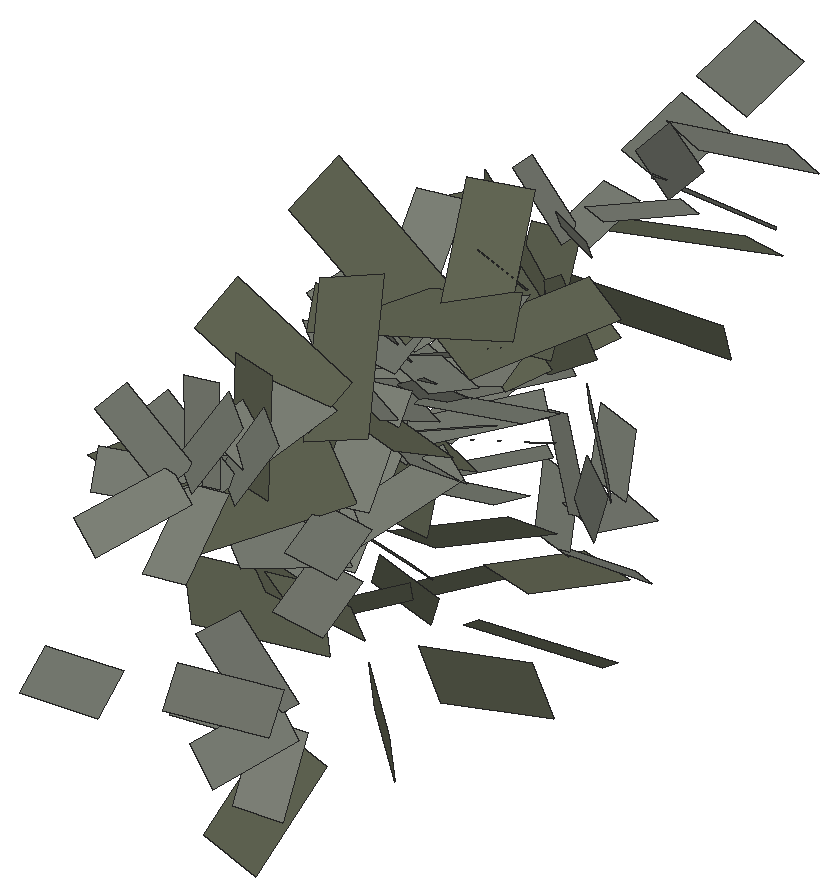
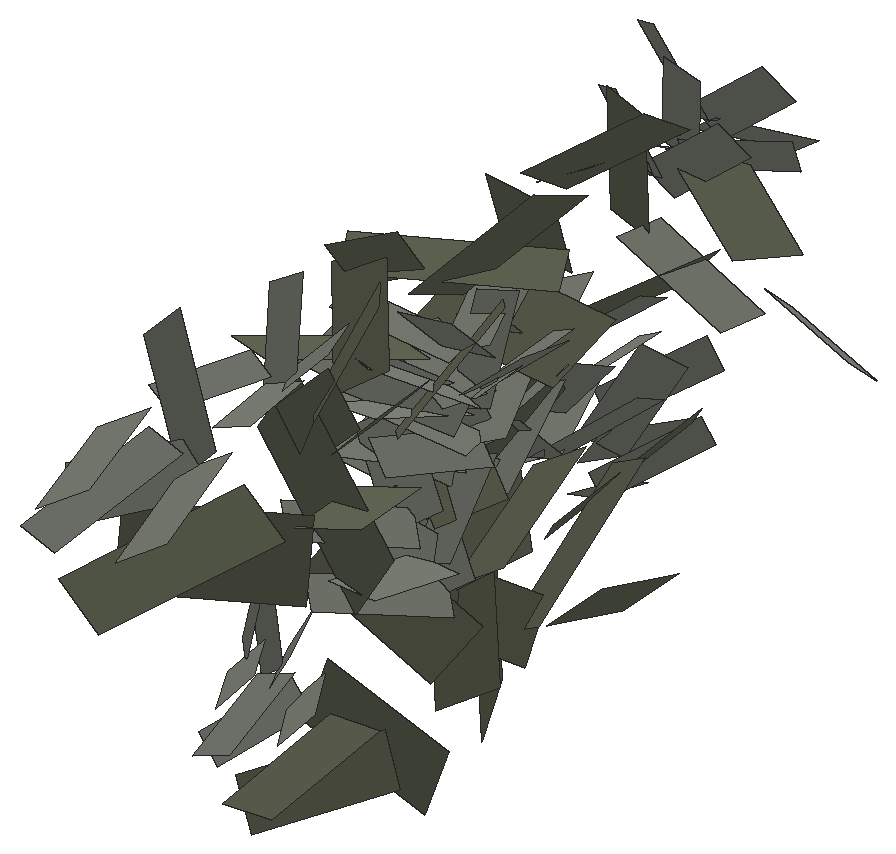
# SketchUp Ruby script. Lengths in inches.
U = 1.inch
M = Sketchup.active_model
def pt(a) = Geom::Point3d.new(a.map { |v| v * U })
def face(e, loops, mat)
  f = e.add_face(loops[0].map { |a| pt(a) })
  loops[1..].each { |l| e.add_face(l.map { |a| pt(a) }).erase! }
  f.material = f.back_material = mat if mat
  f
end
# faces: each face lists its corners as indices into pts; further lists are holes
def faces(e, pts, list, mat = nil) = list.each { |f| face(e, (f[0].is_a?(Array) ? f : [f]).map { |l| l.map { |i| pts[i] } }, mat) }
# xy, xz, yz: faces in a plane at the given z, y or x. An outline is a flat list of corners, or four numbers for a rectangle; further outlines are holes
def ring(l) = l.size == 4 ? [[l[0], l[1]], [l[2], l[1]], [l[2], l[3]], [l[0], l[3]]] : l.each_slice(2).to_a
def flat(e, list, mat, &to3) = list.each { |f| face(e, (f[0].is_a?(Array) ? f : [f]).map { |l| ring(l).map { |u, v| to3.(u, v) } }, mat) }
def xy(e, z, list, mat = nil) = flat(e, list, mat) { |x, y| [x, y, z] }
def xz(e, y, list, mat = nil) = flat(e, list, mat) { |x, z| [x, y, z] }
def yz(e, x, list, mat = nil) = flat(e, list, mat) { |y, z| [x, y, z] }
def lines(e, pts, list) = list.each { |a, b| e.add_line(pt(pts[a]), pt(pts[b])) }
# prism: a flat outline (further loops are holes) pulled along v
def prism(e, loops, v, mat = nil)
  f = face(e, loops, mat); d = Geom::Vector3d.new(v.map { |x| x * U })
  f.pushpull(f.normal.samedirection?(d) ? d.length : -d.length)
end
def box(e, o, s, mat = nil) = prism(e, [[o, [o[0] + s[0], o[1], o[2]], [o[0] + s[0], o[1] + s[1], o[2]], [o[0], o[1] + s[1], o[2]]]], [0, 0, s[2]], mat)
def at(x, y, z, deg = 0) = Geom::Transformation.translation(pt([x, y, z])) * Geom::Transformation.rotation(ORIGIN, Z_AXIS, deg.degrees)
def axes(o, x, y, z) = Geom::Transformation.new([*x, 0, *y, 0, *z, 0, *pt(o).to_a, 1])
def part(name) = M.definitions.add(name)
# library, detail: a bought-in or finely detailed component or shape, given as its bounding box
def library(name, o, s) = part(name).tap { |d| box(d.entities, o, s) }
def detail(e, o, s) = box(e.add_group.entities, o, s)
def put(e, d, t, mat = nil) = e.add_instance(d, t).tap { |i| i.material = mat if mat }
def group(e, t, mat = nil) = e.add_group.tap { |g| g.transformation = t; g.material = mat if mat }.entities
root = M.entities
M.materials.add("viburnumblaasdfas0df1w06d").color = [98, 102, 84]
M.materials.add("viburnumbladsadfasdfad0w122").color = [125, 129, 119]
c1 = part("Component\#315")
p = [[0.25,0,0],[2.05,0.01,0.35],[1.81,4.2,1.66],[0,4.19,1.3125]]
faces(c1.entities,p,[[0,1,2,3]],"viburnumbladsadfasdfad0w122")
c2 = part("viburnumblad2")
put(c2.entities,c1,axes([-19.23,-4.49,-32.18],[83.35428,0,0],[0,79.38502,0],[0,0,83.35428]))
c3 = part("Component\#314")
p = [[0.14,0,0],[2.58,0.05,0.25],[2.44,5.11,2.64],[0,5.05,2.39]]
faces(c3.entities,p,[[0,1,2,3]],"viburnumblaasdfas0df1w06d")
c4 = part("viburnumblad1\#2")
put(c4.entities,c3,axes([-37.25,6.23,19.31],[75.98784,0,0],[0,65.50676,0],[0,0,75.98784]))
put(root,c2,axes([2211.1,274.45,20.97],[0.01246,-0.00054,-0.00182],[0.00031,0.0125,-0.00159],[0.00187,0.00153,0.01237]))
put(root,c4,axes([2212.21,272.84,18.8],[-0.01223,0.00026,0.00635],[-0.0009,-0.01592,-0.0011],[0.0063,-0.0012,0.0122]))
put(root,c2,axes([2213.98,269.82,24.8125],[0.00021,0.01428,-0.00102],[-0.01317,0.00059,0.00559],[0.00561,0.00086,0.01315]))
put(root,c4,axes([2212.88,269.2,15.1],[-0.01278,0.00636,0.00656],[-0.00548,-0.01653,0.00535],[0.00782,0.00178,0.01351]))
put(root,c2,axes([2213.5,271.43,25.38],[-0.01046,0.00558,0.00416],[-0.00525,-0.01025,0.00054],[0.00396,-0.00141,0.01184]))
put(root,c4,axes([2212.19,275.26,23.66],[0.01142,0.00359,-0.00296],[-0.00486,0.01317,-0.00274],[0.00185,0.00298,0.01066]))
put(root,c2,axes([2210.02,261.85,24.99],[-0.00048,-0.01376,-0.00394],[0.01429,-0.00069,0.00066],[-0.00082,-0.00391,0.01375]))
put(root,c4,axes([2213.59,274.42,24.69],[-0.00832,0.00937,0.00389],[-0.0091,-0.01059,0.00604],[0.00643,0.00098,0.01139]))
put(root,c2,axes([2211.89,271.43,27.56],[0.01175,0.00377,-0.00233],[-0.00262,0.01124,0.00497],[0.00358,-0.00416,0.0113]))
put(root,c4,axes([2213.84,275.35,25.35],[0.00125,0.01083,-0.00332],[-0.01199,0.00283,0.0046],[0.00457,0.00236,0.00909]))
put(root,c2,axes([2210.41,254.51,20.4375],[-0.00026,-0.00745,-0.01011],[0.01255,0.00018,-0.00046],[0.00042,-0.01011,0.00745]))
put(root,c2,axes([2213.28,274.3,20.62],[-0.01246,0.00054,0.00182],[0.00014,-0.01079,0.00417],[0.00189,0.00451,0.01162]))
put(root,c4,axes([2210.32,260.4,26.14],[-0.00628,-0.01206,-0.00336],[0.01448,-0.00668,-0.00311],[0.00091,-0.00388,0.01211]))
put(root,c2,axes([2214.56,269.98,22.69],[-0.00958,0.01044,0.00206],[-0.00856,-0.00879,0.00474],[0.00514,0.00211,0.0132]))
put(root,c4,axes([2214.38,265.6875,16.61],[-0.00888,0.00849,0.00791],[-0.01054,-0.01309,0.0022],[0.00721,-0.00377,0.01214]))
put(root,c2,axes([2214.66,264.7,19.88],[-0.00337,0.01279,0.00428],[-0.0107,-0.00403,0.00361],[0.00507,-0.00269,0.01202]))
put(root,c4,axes([2214.9,269.82,27.32],[0.00084,0.01421,0.00442],[-0.01582,-0.0012,0.00687],[0.00595,-0.00438,0.01294]))
put(root,c2,axes([2213.14,272.2,24.1],[-0.01227,-0.00394,0.00243],[0.00307,-0.01072,-0.00188],[0.00284,-0.00132,0.01217]))
put(root,c2,axes([2213.59,271.94,25.17],[-0.01151,-0.00142,0.00146],[0.00195,-0.0101,0.00555],[0.00059,0.0057,0.01018]))
put(root,c2,axes([2211.59,272.02,23.65],[0.00945,-0.00658,0.00199],[0.00631,0.00831,-0.00248],[-0.00002,0.00335,0.01119]))
put(root,c2,axes([2213.35,283.9375,28.75],[0.01049,0.00127,-0.00935],[-0.00649,0.01342,-0.00547],[0.00778,0.00774,0.00978]))
put(root,c2,axes([2211.26,274.54,19.3],[0.00841,-0.00866,0.00086],[0.00975,0.00926,-0.00213],[0.0008,0.00201,0.01242]))
put(root,c2,axes([2214.25,270.37,21.01],[-0.01437,0.00051,0.00412],[0.00025,-0.01266,0.00242],[0.00396,0.00266,0.0135]))
put(root,c2,axes([2211.69,272.4375,26.16],[0.01046,-0.00558,-0.00416],[0.00651,0.0105,0.0023],[0.00246,-0.00407,0.01163]))
put(root,c2,axes([2212.85,274.35,19.14],[-0.00925,-0.00862,0.00362],[0.00803,-0.00772,0.00213],[0.00081,0.00412,0.01188]))
put(root,c4,axes([2212.73,272.77,13.95],[-0.01191,-0.00399,0.00577],[0.00688,-0.0137,0.00471],[0.00376,0.00597,0.01189]))
put(root,c2,axes([2214.6,264.3125,21.46],[0.0065,0.01157,0.00112],[-0.00968,0.00489,0.00566],[0.0049,-0.00389,0.01176]))
put(root,c4,axes([2214.3125,271.3,19.03],[-0.00461,0.01011,0.01059],[-0.01024,-0.0125,0.00748],[0.01168,-0.00415,0.00905]))
put(root,c2,axes([2215.53,256.53,26.72],[-0.00143,0.00635,0.00868],[-0.0108,-0.00196,-0.00037],[0.00136,-0.00839,0.00553]))
put(root,c2,axes([2214.72,255.59,27.625],[0.00668,0.00514,0.00687],[-0.00864,0.00277,0.00603],[0.00109,-0.00897,0.00475]))
put(root,c2,axes([2215.77,263.81,22.85],[-0.00323,0.01225,0.0041],[-0.01189,-0.00447,0.00401],[0.00507,-0.00269,0.01202]))
put(root,c2,axes([2211.75,275.68,22.23],[0.00876,-0.00902,0.0009],[0.00903,0.00857,-0.00197],[0.0008,0.00201,0.01242]))
put(root,c2,axes([2214.05,271.74,27.04],[-0.01175,-0.00377,0.00233],[0.00341,-0.01191,-0.00208],[0.00284,-0.00132,0.01217]))
put(root,c4,axes([2211.4,278.48,20.78],[-0.01053,-0.00014,0.0139],[0.01206,-0.01352,0.00899],[0.00923,0.01297,0.00712]))
put(root,c2,axes([2214.84,277.06,16.86],[0.00461,0.0043,-0.00854],[-0.00856,0.00831,-0.00043],[0.00603,0.00655,0.00655]))
put(root,c2,axes([2215.05,257.75,26.29],[0.00642,0.00493,0.0066],[-0.00933,0.00299,0.00651],[0.00109,-0.00897,0.00475]))
put(root,c4,axes([2215.46,265.77,23.27],[-0.01126,0.00378,0.01091],[-0.00977,-0.0152,-0.00482],[0.00789,-0.0086,0.01113]))
put(root,c4,axes([2212.63,275.59,23.64],[0.00961,-0.00181,-0.00747],[-0.00022,0.01383,-0.00363],[0.00726,0.00235,0.00826]))
put(root,c2,axes([2213.59,265.44,20.49],[0.01096,0.00423,-0.00348],[-0.00277,0.01177,0.00559],[0.00527,-0.00421,0.01149]))
put(root,c2,axes([2215.53,277.53,28.44],[-0.00329,0.00963,-0.00365],[-0.0081,-0.00098,0.00442],[0.00408,0.00455,0.00739]))
put(root,c2,axes([2213,271.33,24.99],[0.01376,-0.00048,-0.00394],[0.00069,0.01429,0.00066],[0.00391,-0.00082,0.01375]))
put(root,c4,axes([2212.2,273.49,21.29],[-0.00859,-0.01039,0.00287],[0.01161,-0.0105,-0.00325],[0.004,0.00034,0.01318]))
put(root,c2,axes([2213.3,275.35,22.07],[-0.00886,-0.00826,0.00347],[0.00892,-0.00858,0.00237],[0.00081,0.00412,0.01188]))
put(root,c4,axes([2215.27,276.48,26.25],[-0.00734,0.00868,0.00063],[-0.0075,-0.00708,0.00798],[0.0058,0.00404,0.00785]))
put(root,c4,axes([2213.09,275.99,14.73],[0.01169,-0.00232,-0.00224],[0.00035,0.01065,-0.00919],[0.00321,0.00758,0.00891]))
put(root,c2,axes([2211.87,273.03,24.6],[0.00292,-0.01119,-0.00341],[0.01302,0.00368,-0.00094],[0.00178,-0.0032,0.01202]))
put(root,c2,axes([2212.29,271.97,22.23],[0.00176,-0.01022,0.00282],[0.01152,0.00195,-0.00013],[-0.00039,0.00304,0.01127]))
put(root,c4,axes([2211.57,269.8,15.05],[0.00317,-0.01127,0.00742],[0.01555,0.00409,-0.00043],[-0.00159,0.00725,0.0117]))
put(root,c2,axes([2213.21,272.23,23.47],[-0.00682,-0.00858,0.00405],[0.00958,-0.00605,0.00332],[-0.00034,0.0052,0.01046]))
put(root,c4,axes([2211.54,282.67,25.5],[0.01385,-0.00786,0.00256],[0.00839,0.01058,-0.01294],[0.00399,0.01072,0.01136]))
put(root,c2,axes([2212.17,275.28,20.5625],[-0.00007,-0.01222,0.00309],[0.01323,-0.00017,-0.00035],[0.00036,0.00309,0.01221]))
put(root,c2,axes([2216.04,264.91,21.22],[-0.01106,0.00576,0.00468],[-0.00631,-0.01247,0.00042],[0.00435,-0.00178,0.01246]))
put(root,c4,axes([2210.71,268.93,25.33],[-0.00321,-0.01557,0.00645],[0.01613,-0.00714,-0.00921],[0.00952,0.00374,0.01377]))
put(root,c2,axes([2216.11,255.57,27.57],[-0.00871,0.00384,0.00541],[-0.00663,-0.00614,-0.00616],[0.00084,-0.00787,0.00624]))
put(root,c4,axes([2216.52,262.4,27.64],[0.00193,0.01121,0.0059],[-0.01433,0.00039,0.00396],[0.00283,-0.0062,0.01085]))
put(root,c2,axes([2212.5625,272.95,24.84],[0.00186,-0.01072,0.00426],[0.01152,0.00195,-0.00013],[-0.00059,0.00423,0.01088]))
put(root,c2,axes([2213.04,272.76,25.83],[-0.00616,-0.01091,-0.00086],[0.01132,-0.00616,-0.00282],[0.00193,-0.00206,0.01224]))
put(root,c2,axes([2215.92,277.65,17.67],[-0.00269,0.008,-0.00714],[-0.00879,0.00257,0.00619],[0.00614,0.00718,0.00574]))
put(root,c4,axes([2211.95,274.06,16.04],[-0.00313,-0.01186,0.00638],[0.01559,-0.00367,0.00082],[0.00085,0.00636,0.01225]))
put(root,c2,axes([2215.42,270.81,24.33],[-0.01376,0.00048,0.00394],[0.00028,-0.01406,0.00269],[0.00396,0.00266,0.0135]))
put(root,c2,axes([2214.72,286.47,31.09],[0.01093,0.00132,-0.00974],[-0.00601,0.01242,-0.00506],[0.00778,0.00774,0.00978]))
put(root,c2,axes([2216.15,260.37,15.79],[-0.00143,0.00682,0.00818],[-0.0095,-0.00594,0.0033],[0.00662,-0.0068,0.00682]))
put(root,c4,axes([2214.77,275.03,24.56],[0.00373,0.00907,-0.00579],[-0.00694,0.00792,0.00773],[0.00862,0.00055,0.00603]))
put(root,c4,axes([2214.86,264.57,12.95],[-0.00935,-0.00415,0.00773],[-0.00246,-0.01147,-0.00913],[0.00851,-0.00702,0.00652]))
put(root,c4,axes([2213.29,270.85,17.48],[-0.01204,-0.00702,0.00725],[0.00958,-0.01547,0.00093],[0.0058,0.00442,0.01392]))
put(root,c2,axes([2214.66,278.24,28.47],[0.00829,0.00118,-0.00446],[-0.00277,0.00969,-0.0025],[0.00431,0.00339,0.00782]))
put(root,c4,axes([2215.11,263.97,25.74],[0.01317,0.00353,0.00249],[-0.00497,0.01356,0.00706],[-0.00054,-0.00655,0.0122]))
put(root,c2,axes([2215.8,278.98,18.64],[0.0048,0.00448,-0.0089],[-0.00793,0.0077,-0.0004],[0.00603,0.00655,0.00655]))
put(root,c2,axes([2214.54,264.77,23.46],[0.01242,0.00411,-0.00252],[-0.00277,0.01177,0.00559],[0.00395,-0.00468,0.01183]))
put(root,c4,axes([2211.09,268.5625,28.48],[0.00835,-0.01477,-0.00252],[0.01522,0.00998,-0.00805],[0.00724,0.00145,0.01548]))
put(root,c2,axes([2212.88,272.67,27.58],[0.00304,-0.01166,-0.00355],[0.01206,0.00341,-0.00087],[0.00178,-0.0032,0.01202]))
put(root,c2,axes([2214.62,257.03,27.39],[0.01089,0.00092,0.00104],[-0.00149,0.00552,0.00975],[0.0002,-0.00927,0.00435]))
put(root,c4,axes([2212.52,275.31,12.66],[0.00779,-0.00697,0.00615],[0.01029,0.00367,-0.00887],[0.00279,0.00941,0.00713]))
put(root,c4,axes([2211.3125,281.45,22.77],[0.0041,-0.00986,0.01208],[0.01717,-0.00172,-0.00723],[0.00492,0.01267,0.00868]))
put(root,c4,axes([2214.62,260.45,25.71],[0.0117,-0.0027,-0.00014],[0.00141,0.00653,0.01192],[-0.00257,-0.00994,0.00471]))
put(root,c2,axes([2212.92,271.86,23.09],[0.00958,-0.01044,-0.00206],[0.01029,0.0098,-0.00181],[0.00273,-0.00027,0.01406]))
put(root,c4,axes([2214.4375,276.06,26.65],[-0.01002,-0.00367,0.00577],[0.0058,-0.01266,0.00203],[0.00466,0.00382,0.01053]))
put(root,c4,axes([2213.39,269.71,11.49],[-0.00616,-0.00011,0.01357],[0.00475,-0.0165,0.00202],[0.01294,0.00445,0.00591]))
put(root,c4,axes([2212.73,273.41,10.77],[-0.00376,-0.0039,0.01194],[0.01323,-0.00731,0.00178],[0.00528,0.01082,0.0052]))
put(root,c2,axes([2214.99,278.45,17.4375],[0.00948,-0.00167,-0.00544],[-0.00216,0.00929,-0.00661],[0.00531,0.00641,0.00728]))
put(root,c2,axes([2215.59,266.12,19.93],[-0.01192,-0.00395,0.00242],[0.00393,-0.01356,-0.00276],[0.00316,-0.0017,0.01283]))
put(root,c2,axes([2216.06,259.32,16.96],[0.00667,0.00821,0.00496],[-0.00717,0.00016,0.00937],[0.00645,-0.00831,0.00509]))
put(root,c2,axes([2214.46,271.66,22.625],[-0.00988,-0.00976,0.00351],[0.01049,-0.01076,-0.00039],[0.00277,0.00219,0.01388]))
put(root,c2,axes([2213.94,285.78,29.32],[0.01262,-0.00712,-0.00249],[0.00385,0.01054,-0.01059],[0.00659,0.00804,0.0104]))
put(root,c2,axes([2213.13,271.8,21.19],[-0.0002,-0.01371,0.00098],[0.01527,-0.0004,-0.00242],[0.00226,0.00098,0.01411]))
put(root,c2,axes([2216.97,262.77,28.64],[-0.01426,0.00099,0.00559],[-0.00302,-0.01157,-0.00566],[0.00428,-0.00706,0.01216]))
put(root,c4,axes([2215.85,270.37,28.07],[0.00971,0.0077,-0.00377],[-0.00736,0.01191,0.00523],[0.00557,-0.00177,0.01033]))
put(root,c2,axes([2215.24,284.22,27.28],[-0.0106,-0.00225,0.00809],[0.00771,-0.01018,0.00728],[0.00487,0.01032,0.00927]))
put(root,c2,axes([2217.04,278.6,18.11],[-0.0086,0.00684,-0.0012],[-0.00415,-0.00354,0.00962],[0.00557,0.00793,0.00532]))
put(root,c2,axes([2216.55,257.11,27.49],[-0.01089,-0.00092,-0.00104],[0.00144,-0.00742,-0.00803],[-0.00015,-0.00772,0.00646]))
put(root,c2,axes([2217.42,258.43,17.37],[-0.00083,0.00664,0.00958],[-0.0095,-0.00594,0.0033],[0.00675,-0.00756,0.00582]))
put(root,c2,axes([2214.16,266.03,22.08],[0.01106,-0.00576,-0.00468],[0.00696,0.01121,0.00265],[0.00276,-0.0046,0.01219]))
put(root,c2,axes([2214.62,278.08,15.92],[0.00898,-0.00714,0.00125],[0.00484,0.00482,-0.00724],[0.0044,0.00684,0.00749]))
put(root,c2,axes([2213.87,285.03,27.32],[0.00722,-0.01189,0.00649],[0.01053,0.00219,-0.0077],[0.0056,0.00897,0.01021]))
put(root,c2,axes([2216.18,278.43,27.74],[-0.00905,-0.00157,0.00381],[0.00376,-0.00932,0.00479],[0.00255,0.00548,0.00745]))
put(root,c2,axes([2217.49,260.04,16.58],[-0.00784,0.00117,0.00859],[-0.00546,-0.0084,-0.00383],[0.00631,-0.00716,0.00674]))
put(root,c2,axes([2214.78,256.4,28.73],[0.00871,-0.00384,-0.00541],[0.00664,0.00406,0.00749],[-0.00079,-0.00912,0.00457]))
put(root,c2,axes([2214.99,258.54,27.42],[0.00909,-0.00401,-0.00564],[0.00597,0.00365,0.00674],[-0.00079,-0.00912,0.00457]))
put(root,c2,axes([2215.08,279.4,29],[0.00889,-0.00537,-0.00033],[0.00481,0.00824,-0.00432],[0.00239,0.00342,0.00851]))
put(root,c2,axes([2216.93,261.29,16.16],[-0.01071,-0.0052,0.00268],[0.00135,-0.00683,-0.00788],[0.0054,-0.00736,0.0073]))
put(root,c2,axes([2216.82,265.12,22.89],[-0.01242,-0.00411,0.00252],[0.00364,-0.01255,-0.00256],[0.00316,-0.0017,0.01283]))
put(root,c2,axes([2216.69,278.09,16.5625],[-0.00948,0.00167,0.00544],[0.00331,-0.00711,0.00795],[0.00466,0.00836,0.00554]))
put(root,c2,axes([2214.4375,272.32,24.51],[-0.00021,-0.01428,0.00102],[0.01414,-0.00037,-0.00224],[0.00226,0.00098,0.01411]))
put(root,c4,axes([2214.45,271.63,26.14],[0.01206,-0.00628,-0.00336],[0.00668,0.01448,-0.00311],[0.00388,0.00091,0.01211]))
